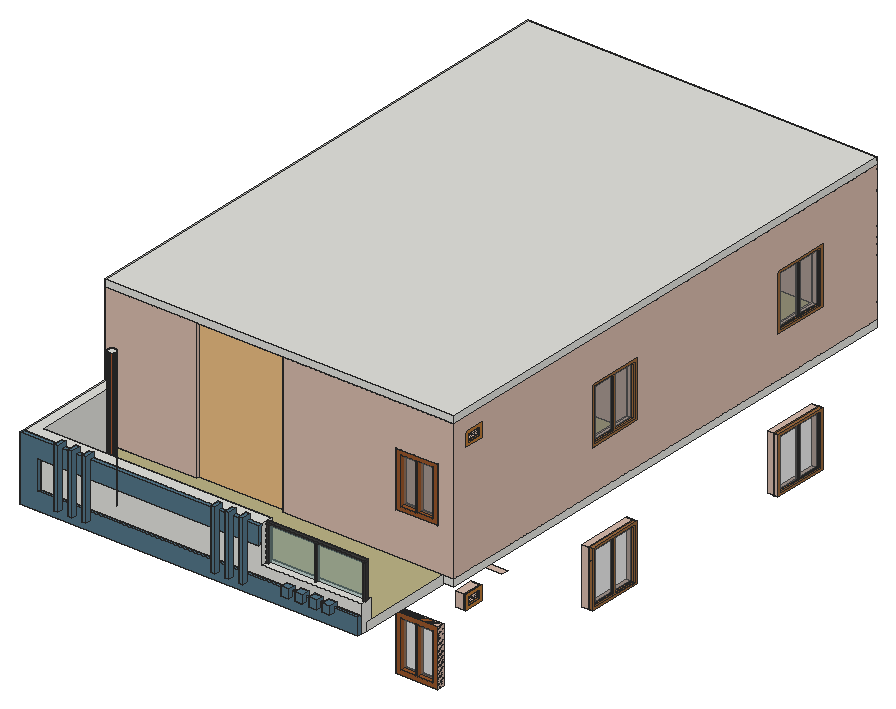
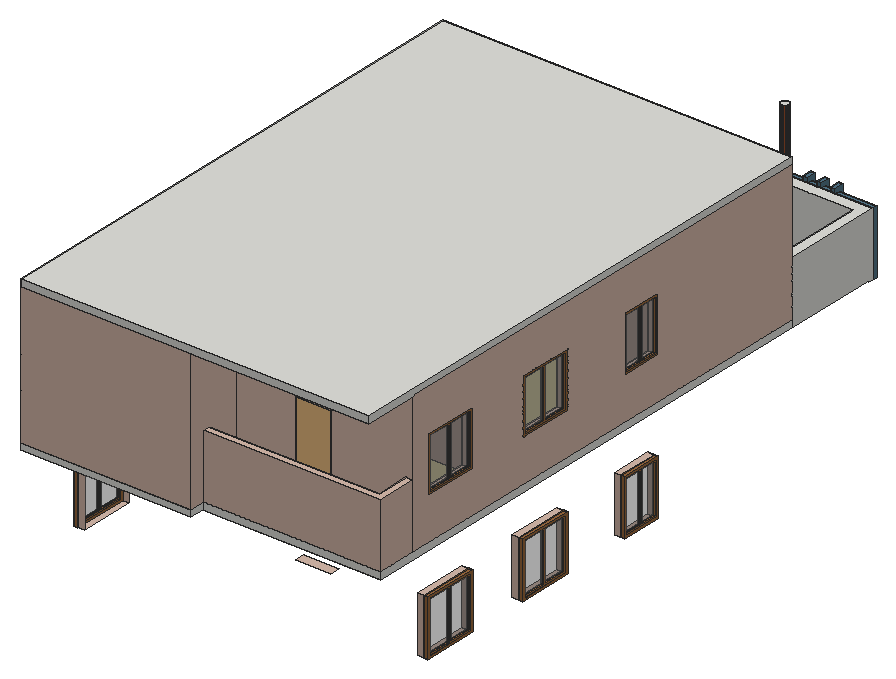
# SketchUp Ruby script. Lengths in inches.
U = 1.inch
M = Sketchup.active_model
def pt(a) = Geom::Point3d.new(a.map { |v| v * U })
def face(e, loops, mat)
  f = e.add_face(loops[0].map { |a| pt(a) })
  loops[1..].each { |l| e.add_face(l.map { |a| pt(a) }).erase! }
  f.material = f.back_material = mat if mat
  f
end
# faces: each face lists its corners as indices into pts; further lists are holes
def faces(e, pts, list, mat = nil) = list.each { |f| face(e, (f[0].is_a?(Array) ? f : [f]).map { |l| l.map { |i| pts[i] } }, mat) }
# xy, xz, yz: faces in a plane at the given z, y or x. An outline is a flat list of corners, or four numbers for a rectangle; further outlines are holes
def ring(l) = l.size == 4 ? [[l[0], l[1]], [l[2], l[1]], [l[2], l[3]], [l[0], l[3]]] : l.each_slice(2).to_a
def flat(e, list, mat, &to3) = list.each { |f| face(e, (f[0].is_a?(Array) ? f : [f]).map { |l| ring(l).map { |u, v| to3.(u, v) } }, mat) }
def xy(e, z, list, mat = nil) = flat(e, list, mat) { |x, y| [x, y, z] }
def xz(e, y, list, mat = nil) = flat(e, list, mat) { |x, z| [x, y, z] }
def yz(e, x, list, mat = nil) = flat(e, list, mat) { |y, z| [x, y, z] }
def lines(e, pts, list) = list.each { |a, b| e.add_line(pt(pts[a]), pt(pts[b])) }
# prism: a flat outline (further loops are holes) pulled along v
def prism(e, loops, v, mat = nil)
  f = face(e, loops, mat); d = Geom::Vector3d.new(v.map { |x| x * U })
  f.pushpull(f.normal.samedirection?(d) ? d.length : -d.length)
end
def box(e, o, s, mat = nil) = prism(e, [[o, [o[0] + s[0], o[1], o[2]], [o[0] + s[0], o[1] + s[1], o[2]], [o[0], o[1] + s[1], o[2]]]], [0, 0, s[2]], mat)
def at(x, y, z, deg = 0) = Geom::Transformation.translation(pt([x, y, z])) * Geom::Transformation.rotation(ORIGIN, Z_AXIS, deg.degrees)
def axes(o, x, y, z) = Geom::Transformation.new([*x, 0, *y, 0, *z, 0, *pt(o).to_a, 1])
def part(name) = M.definitions.add(name)
# library, detail: a bought-in or finely detailed component or shape, given as its bounding box
def library(name, o, s) = part(name).tap { |d| box(d.entities, o, s) }
def detail(e, o, s) = box(e.add_group.entities, o, s)
def put(e, d, t, mat = nil) = e.add_instance(d, t).tap { |i| i.material = mat if mat }
def group(e, t, mat = nil) = e.add_group.tap { |g| g.transformation = t; g.material = mat if mat }.entities
root = M.entities
M.materials.add("TEAKcrown-cut").color = [186, 122, 55]
M.materials.add("[0027_PeachPuff]").color = [83, 118, 137]
M.materials.add("[0042_Sienna]").color = [160, 82, 45]
M.materials.add("[Color B01]").color = [216, 187, 172]
M.materials.add("[Color E03]").color = [255, 255, 101]
M.materials.add("[Color E05]").color = [255, 255, 0]
M.materials.add("[Color M07]").color = [58, 58, 58]
M.materials.add("[Tile Ceramic Natural]").color = [189, 180, 134]
M.materials.add("[Translucent Glass Blue]").color = [141, 178, 174]
M.materials["[Translucent Glass Blue]"].alpha = 0.5
M.materials.add("[Translucent Glass Gray]").color = [128, 128, 128]
M.materials["[Translucent Glass Gray]"].alpha = 0.5
M.materials.add("[Translucent_Glass_Gray]3").color = [255, 255, 255]
M.materials["[Translucent_Glass_Gray]3"].alpha = 0.5
M.materials.add("[Wood Bamboo]").color = [122, 73, 29]
M.materials.add("[Wood Cherry Original]").color = [152, 86, 42]
M.materials.add("[Wood Floor]").color = [155, 105, 61]
c1 = part("window full")
xy(c1.entities,0,[[0,0,14.17,66.54]])
xy(c1.entities,2.26,[[12.2,2.26,14.17,64.28]],"[Wood Floor]")
xy(c1.entities,2.36,[[0,2.36,1.97,64.17]],"[Wood Floor]")
xy(c1.entities,3.74,[[11.42,3.74,12.2,32.875],[11.42,33.66,12.2,62.79]],"[Wood Floor]")
xy(c1.entities,3.9375,[[1.97,3.9375,2.76,32.77],[1.97,33.76,2.76,62.6]],"[Wood Floor]")
xy(c1.entities,4.18,[[2.76,4.18,11.42,32.09],[2.76,34.45,11.42,62.35]],"[Wood Floor]")
xy(c1.entities,69.83,[[2.76,4.18,11.42,32.09],[2.76,34.45,11.42,62.35]],"[Wood Floor]")
xy(c1.entities,70.08,[[1.97,3.9375,2.76,32.77],[1.97,33.76,2.76,62.6]])
xy(c1.entities,70.27,[[11.42,32.875,12.2,33.66]])
xy(c1.entities,70.27,[[11.42,3.74,12.2,32.875],[11.42,33.66,12.2,62.79]],"[Wood Floor]")
xy(c1.entities,71.65,[[0,2.36,1.97,64.17]])
xy(c1.entities,71.76,[[12.2,2.26,14.17,64.28]],"[Wood Floor]")
xy(c1.entities,74.02,[[0,0,14.17,66.54]],"[Wood Floor]")
xz(c1.entities,0,[[0,0,14.17,74.02]],"[Wood Floor]")
xz(c1.entities,2.26,[[12.2,2.26,14.17,71.76]],"[Wood Floor]")
xz(c1.entities,2.36,[[0,2.36,1.97,71.65]],"[Wood Floor]")
xz(c1.entities,3.74,[[11.42,3.74,12.2,70.27]],"[Wood Floor]")
xz(c1.entities,3.9375,[[1.97,3.9375,2.76,70.08]],"[Wood Floor]")
xz(c1.entities,4.18,[[2.76,4.18,11.42,69.83]],"[Wood Floor]")
xz(c1.entities,32.09,[[2.76,4.18,11.42,69.83]],"[Wood Floor]")
xz(c1.entities,32.77,[[1.97,3.9375,2.76,70.08]],"[Wood Floor]")
xz(c1.entities,32.875,[[11.42,3.74,12.2,70.27]],"[Wood Floor]")
xz(c1.entities,33.66,[[11.42,3.74,12.2,47.88],[11.42,47.88,12.2,70.27]],"[Wood Floor]")
xz(c1.entities,33.76,[[1.97,3.9375,2.76,70.08]],"[Wood Floor]")
xz(c1.entities,34.45,[[2.76,4.18,11.42,69.83]],"[Wood Floor]")
xz(c1.entities,62.35,[[2.76,4.18,11.42,69.83]],"[Wood Floor]")
xz(c1.entities,62.6,[[1.97,3.9375,2.76,70.08]],"[Wood Floor]")
xz(c1.entities,62.79,[[11.42,3.74,12.2,70.27]],"[Wood Floor]")
xz(c1.entities,64.17,[[0,2.36,1.97,71.65]],"[Wood Floor]")
xz(c1.entities,64.28,[[12.2,2.26,14.17,71.76]],"[Wood Floor]")
xz(c1.entities,66.54,[[0,0,14.17,74.02]],"[Wood Floor]")
yz(c1.entities,0,[[[0,0,66.54,74.02],[2.36,2.36,64.17,71.65]]],"[Wood Floor]")
yz(c1.entities,1.97,[[[2.36,2.36,64.17,71.65],[3.9375,3.9375,32.77,70.08],[33.76,3.9375,62.6,70.08]]],"[Wood Floor]")
yz(c1.entities,2.76,[[32.77,3.9375,33.76,4.18],[32.77,4.18,33.76,69.83],[32.77,69.83,33.76,70.08]])
yz(c1.entities,2.76,[[[3.9375,3.9375,32.77,70.08],[4.18,4.18,32.09,69.83]],[[33.76,3.9375,62.6,70.08],[34.45,4.18,62.35,69.83]]],"[Wood Floor]")
yz(c1.entities,11.42,[[32.875,69.83,33.66,70.27]])
yz(c1.entities,11.42,[[[3.74,3.74,32.875,70.27],[4.18,4.18,32.09,69.83]],[[33.66,3.74,62.79,70.27],[34.45,4.18,62.35,69.83]]],"[Wood Floor]")
yz(c1.entities,12.2,[[[2.26,2.26,64.28,71.76],[3.74,3.74,32.875,70.27],[33.66,3.74,62.79,70.27]]],"[Wood Floor]")
yz(c1.entities,14.17,[[[0,0,66.54,74.02],[2.26,2.26,64.28,71.76]]],"[Wood Floor]")
p = [[11.42,32.875,70.27],[11.42,32.875,70.28],[11.42,32.875,69.83],[11.42,32.09,69.83],[11.42,34.45,69.83],[11.42,33.66,69.83]]
lines(c1.entities,p,[[0,1],[2,3],[4,5]])
c2 = part("Group\#7")
g1 = group(c2.entities,at(1.67,3.02,2.71))
yz(g1,0,[[0,0,20.13,42.58]],"[Translucent Glass Gray]")
g2 = group(c2.entities,at(0,0,0))
put(g2,c1,axes([0,0,0],[0.2352,0,0],[0,0.72142,0],[0,0,0.64851]))
g3 = group(g2,at(1.67,24.85,2.71))
yz(g3,0,[[0,0,20.13,42.58]],"[Translucent Glass Gray]")
c3 = part("Group30\#1")
xy(c3.entities,0,[[-14.0625,-20.0625,-0.59,20.0625],[0.59,-20.0625,14.0625,20.0625]],"[Translucent Glass Gray]")
c4 = part("Group29\#1")
prism(c4.entities,[[[-18,24,0],[18,24,0],[18,-24,0],[-18,-24,0]],[[14.0625,20.0625,0],[0.59,20.0625,0],[0.59,-20.0625,0],[14.0625,-20.0625,0]],[[-0.59,20.0625,0],[-14.0625,20.0625,0],[-14.0625,-20.0625,0],[-0.59,-20.0625,0]]],[0,0,5.875],"[Wood Cherry Original]")
put(c4.entities,c3,at(0,0,2.9375))
c5 = part("Component\#10")
box(c5.entities,[0,0,0],[19,0.25,3.7],"[Translucent_Glass_Gray]3")
c6 = part("Ventilation_window")
g4 = group(c6.entities,at(-76.91,6.38,0),"TEAKcrown-cut")
xy(g4,-1.7,[[0,0,24,3]])
xy(g4,2.5,[[2.5,0,21.5,3]])
xy(g4,17.5,[[2.5,0,21.5,3]])
xy(g4,21.7,[[0,0,24,3]])
xz(g4,0,[[[0,-1.7,24,21.7],[2.5,2.5,21.5,17.5]]],"TEAKcrown-cut")
xz(g4,3,[[[0,-1.7,24,21.7],[2.5,2.5,21.5,17.5]]])
yz(g4,0,[[0,-1.7,3,21.7]])
yz(g4,2.5,[[0,2.5,3,2.5,3,4.31,0,6.48],[3,4.31,3,17.5,0,17.5,0,6.48]])
yz(g4,21.5,[[0,2.5,3,17.5]])
yz(g4,24,[[0,-1.7,3,21.7]])
put(g4,c5,axes([2.5,3.14,11.94],[1,0,0],[0,0.58779,0.80902],[0,-0.80902,0.58779]))
put(g4,c5,axes([2.5,3.16,14.6],[1,0,0],[0,0.58779,0.80902],[0,-0.80902,0.58779]))
put(g4,c5,axes([2.5,3,4.31],[1,0,0],[0,0.58779,0.80902],[0,-0.80902,0.58779]))
put(g4,c5,axes([2.5,3.14,9.46],[1,0,0],[0,0.58779,0.80902],[0,-0.80902,0.58779]))
put(g4,c5,axes([2.5,2.99,7.08],[1,0,0],[0,0.58779,0.80902],[0,-0.80902,0.58779]))
c7 = part("Group70\#1")
box(c7.entities,[313.8,73.72,268.25],[1.18,2.36,29.23])
c8 = part("Group69\#1")
box(c8.entities,[356.12,73.72,268.25],[2.36,2.36,29.23])
c9 = part("Group71\#1")
box(c9.entities,[270.3,73.52,297.48],[88.18,2.76,1.77])
c10 = part("Group68\#1")
box(c10.entities,[270.3,73.72,268.25],[2.37,2.36,29.23])
c11 = part("Group74\#1")
xz(c11.entities,74.9,[[271.49,268.25,357.3,297.48]],"[Translucent Glass Blue]")
c12 = part("Group\#12")
put(c12.entities,c7,at(-270.3,-73.52,-268.25),"[Color M07]")
put(c12.entities,c8,at(-270.3,-73.52,-268.25),"[Color M07]")
put(c12.entities,c9,at(-270.3,-73.52,-268.25),"[Color M07]")
put(c12.entities,c10,at(-270.3,-73.52,-268.25),"[Color M07]")
put(c12.entities,c11,at(-270.3,-73.52,-268.25))
c13 = part("Component\#9")
xy(c13.entities,0,[[[0,0,6.875,4],[0.7,0.7,6.17,3.3]]],"[Color E05]")
xy(c13.entities,0.625,[[0.7,0.7,6.17,3.3]],"[Color E05]")
xy(c13.entities,4.5625,[[0,4,6.875,6.6875]])
xy(c13.entities,7.25,[[0,0,6.875,6.6875]],"[0027_PeachPuff]")
xz(c13.entities,0,[[0,0,6.875,7.25]],"[0027_PeachPuff]")
xz(c13.entities,0.7,[[0.7,0,6.17,0.625]])
xz(c13.entities,3.3,[[0.7,0,6.17,0.625]],"[Color E05]")
xz(c13.entities,4,[[0,0,6.875,4.5625]])
xz(c13.entities,6.6875,[[0,4.5625,6.875,7.25]])
yz(c13.entities,0,[[0,0,0,7.25,6.6875,7.25,6.6875,4.5625,4,4.5625,4,0]],"[0027_PeachPuff]")
yz(c13.entities,0.7,[[0.7,0,3.3,0.625]],"[Color E05]")
yz(c13.entities,6.17,[[0.7,0,3.3,0.625]],"[Color E05]")
yz(c13.entities,6.875,[[0,0,4,0,4,4.5625,6.6875,4.5625,6.6875,7.25,0,7.25]],"[0027_PeachPuff]")
c14 = part("Vertical support post")
prism(c14.entities,[[[3.5625,0,-4],[3.5625,0,43.375],[3.5625,4,43.375],[3.5625,4,47.375],[3.5625,-4,47.375],[3.5625,-4,-4]]],[-3.5625,0,0],"[0027_PeachPuff]")
c15 = library("door by lz",[5.91,-4.92,0],[35.43,6.61,78.74])
c16 = part("Union")
xy(c16.entities,0,[[0,87.5,0,494.5,71.05,494.5,71.05,485.5,9,485.5,9,387.5,117,387.5,117,381.5,9,381.5,9,213.5,113.3,213.5,113.3,207.5,9,207.5,9,96.5,78.6875,96.5,78.6875,87.5],[[153,87.5,153,93.5,239,93.5,239,171.5,153,171.5,153,207.5,143.3,207.5,143.3,213.5,153,213.5,153,286.45,159,286.45,159,177.5,250.23,177.5,250.23,171.5,245,171.5,245,93.5,291,93.5,291,171.5,274.23,171.5,274.23,177.5,291,177.5,291,321.5,159,321.5,159,316.45,153,316.45,153,347.3125,159,347.3125,159,327.5,246,327.5,246,383.5,159,383.5,159,389.5,291,389.5,291,533.5,159,533.5,159,424.27,153,424.27,153,431.5,144.37,431.5,144.37,437.5,153,437.5,153,485.5,117,485.5,117,437.5,124.37,437.5,124.37,431.5,117,431.5,117,424.23,111,424.23,111,485.5,101.05,485.5,101.05,494.5,153,494.5,153,542.5,300,542.5,300,87.5],[252,327.5,291,383.5]],[153,377.3125,158.97,394.27],[111,387.5,117,394.27]])
xy(c16.entities,36,[[250.39,87.5,286.39,93.5],[0,230.6875,9,266.6875],[291,236.77,300,284.77],[0,328.61,9,376.61],[0,430.49,9,478.49],
  [291,436.51,300,484.51]])
xy(c16.entities,84,[[250.39,87.5,286.39,93.5],[250.23,171.5,274.23,177.5],[113.3,207.5,143.3,213.5],[0,230.6875,9,266.6875],[291,236.77,300,284.77],
  [153,286.45,159,316.45],[0,328.61,9,376.61],[153,347.3125,158.97,377.3125],[111,394.27,117,424.23],[153,394.27,159,424.27],
  [0,430.49,9,478.49],[124.37,431.5,144.37,437.5],[291,436.51,300,484.51],[71.05,485.5,101.05,494.5]])
xy(c16.entities,96,[[291,100.54,300,117.47]])
xy(c16.entities,108,[[291,100.54,300,117.47]])
xy(c16.entities,120,[[[0,87.5,78.6875,87.5,78.6875,96.5,9,96.5,9,207.5,153,207.5,153,171.5,239,171.5,239,93.5,153,93.5,153,87.5,300,87.5,300,542.5,153,542.5,153,494.5,0,494.5],[9,213.5,9,381.5,117,381.5,117,431.5,153,431.5,153,213.5],[159,327.5,159,347.3125,158.97,347.3125,158.97,394.27,159,394.27,159,533.5,291,533.5,291,389.5,159,389.5,159,383.5,246,383.5,246,327.5],[159,177.5,291,321.5],[9,387.5,111,485.5],[245,93.5,291,171.5],[252,327.5,291,383.5],[117,437.5,153,485.5]]])
xz(c16.entities,87.5,[[0,0,78.6875,120],[[153,0,300,120],[250.39,36,286.39,84]]],"[Color B01]")
xz(c16.entities,93.5,[[153,0,239,120],[[245,0,291,120],[250.39,36,286.39,84]]])
xz(c16.entities,96.5,[[9,0,78.6875,120]])
xz(c16.entities,100.54,[[291,96,300,108]])
xz(c16.entities,117.47,[[291,96,300,108]])
xz(c16.entities,171.5,[[153,0,239,120],[245,0,250.23,0,250.23,84,274.23,84,274.23,0,291,0,291,120,245,120]],"[Color B01]")
xz(c16.entities,177.5,[[159,0,159,120,291,120,291,0,274.23,0,274.23,84,250.23,84,250.23,0]])
xz(c16.entities,207.5,[[9,0,113.3,0,113.3,84,143.3,84,143.3,0,153,0,153,120,9,120]],"[Color B01]")
xz(c16.entities,213.5,[[9,0,113.3,120],[143.3,0,143.3,84,113.3,84,113.3,120,153,120,153,0]])
xz(c16.entities,230.6875,[[0,36,9,84]])
xz(c16.entities,236.77,[[291,36,300,84]])
xz(c16.entities,266.6875,[[0,36,9,84]])
xz(c16.entities,284.77,[[291,36,300,84]])
xz(c16.entities,286.45,[[153,0,159,84]])
xz(c16.entities,316.45,[[153,0,159,84]])
xz(c16.entities,321.5,[[159,0,291,120]],"[Color B01]")
xz(c16.entities,327.5,[[159,0,246,120],[252,0,291,120]])
xz(c16.entities,328.61,[[0,36,9,84]])
xz(c16.entities,347.3125,[[153,0,153,84,158.97,84,158.97,120,159,120,159,0]])
xz(c16.entities,376.61,[[0,36,9,84]])
xz(c16.entities,377.3125,[[153,0,158.97,84]])
xz(c16.entities,381.5,[[9,0,117,120]],"[Color B01]")
xz(c16.entities,383.5,[[252,0,291,120]])
xz(c16.entities,383.5,[[159,0,246,120]],"[Color B01]")
xz(c16.entities,387.5,[[9,0,111,120]])
xz(c16.entities,389.5,[[159,0,291,120]])
xz(c16.entities,394.27,[[111,0,117,84],[153,0,158.97,84],[158.97,84,159,120]])
xz(c16.entities,424.23,[[111,0,117,84]])
xz(c16.entities,424.27,[[153,0,159,84]])
xz(c16.entities,430.49,[[0,36,9,84]])
xz(c16.entities,431.5,[[117,0,124.37,0,124.37,84,144.37,84,144.37,0,153,0,153,120,117,120]],"[Color B01]")
xz(c16.entities,436.51,[[291,36,300,84]])
xz(c16.entities,437.5,[[117,0,117,120,153,120,153,0,144.37,0,144.37,84,124.37,84,124.37,0]])
xz(c16.entities,478.49,[[0,36,9,84]])
xz(c16.entities,484.51,[[291,36,300,84]])
xz(c16.entities,485.5,[[117,0,153,120]])
xz(c16.entities,485.5,[[9,0,71.05,0,71.05,84,101.05,84,101.05,0,111,0,111,120,9,120]],"[Color B01]")
xz(c16.entities,494.5,[[0,0,0,120,153,120,153,0,101.05,0,101.05,84,71.05,84,71.05,0]])
xz(c16.entities,533.5,[[159,0,291,120]],"[Color B01]")
xz(c16.entities,542.5,[[153,0,300,120]])
yz(c16.entities,0,[[[87.5,0,494.5,120],[430.49,36,478.49,84],[328.61,36,376.61,84],[230.6875,36,266.6875,84]]],"[Color B01]")
yz(c16.entities,9,[[96.5,0,207.5,120],[[213.5,0,381.5,120],[328.61,36,376.61,84],[230.6875,36,266.6875,84]],[[387.5,0,485.5,120],[430.49,36,478.49,84]]])
yz(c16.entities,71.05,[[485.5,0,494.5,84]])
yz(c16.entities,78.6875,[[87.5,0,96.5,120]])
yz(c16.entities,101.05,[[485.5,0,494.5,84]])
yz(c16.entities,111,[[387.5,0,387.5,120,485.5,120,485.5,0,424.23,0,424.23,84,394.27,84,394.27,0]])
yz(c16.entities,113.3,[[207.5,0,213.5,84]])
yz(c16.entities,117,[[381.5,0,394.27,0,394.27,84,424.23,84,424.23,0,431.5,0,431.5,120,381.5,120],[437.5,0,485.5,120]])
yz(c16.entities,124.37,[[431.5,0,437.5,84]])
yz(c16.entities,143.3,[[207.5,0,213.5,84]])
yz(c16.entities,144.37,[[431.5,0,437.5,84]])
yz(c16.entities,153,[[87.5,0,93.5,120],[437.5,0,485.5,120],[494.5,0,542.5,120]])
yz(c16.entities,153,[[171.5,0,207.5,120],[213.5,0,213.5,120,431.5,120,431.5,0,424.27,0,424.27,84,394.27,84,394.27,0,377.3125,0,377.3125,84,347.3125,84,347.3125,0,316.45,0,316.45,84,286.45,84,286.45,0]],"[Color B01]")
yz(c16.entities,158.97,[[377.3125,0,394.27,0,394.27,120,347.3125,120,347.3125,84,377.3125,84]])
yz(c16.entities,159,[[327.5,0,347.3125,120],[383.5,0,389.5,120],[424.27,0,533.5,0,533.5,120,394.27,120,394.27,84,424.27,84]])
yz(c16.entities,159,[[177.5,0,286.45,0,286.45,84,316.45,84,316.45,0,321.5,0,321.5,120,177.5,120]],"[Color B01]")
yz(c16.entities,239,[[93.5,0,171.5,120]])
yz(c16.entities,245,[[93.5,0,171.5,120]])
yz(c16.entities,246,[[327.5,0,383.5,120]])
yz(c16.entities,250.23,[[171.5,0,177.5,84]])
yz(c16.entities,250.39,[[87.5,36,93.5,84]])
yz(c16.entities,252,[[327.5,0,383.5,120]])
yz(c16.entities,274.23,[[171.5,0,177.5,84]])
yz(c16.entities,286.39,[[87.5,36,93.5,84]])
yz(c16.entities,291,[[[93.5,0,171.5,120],[100.54,96,117.47,108]],[[177.5,0,321.5,120],[236.77,36,284.77,84]],[327.5,0,383.5,120],[[389.5,0,533.5,120],[436.51,36,484.51,84]]])
yz(c16.entities,300,[[[87.5,0,542.5,120],[436.51,36,484.51,84],[236.77,36,284.77,84],[100.54,96,117.47,108]]],"[Color B01]")
put(c16.entities,c15,axes([153.59,321.46,0],[0,-0.84667,0],[0.14881,0,0],[0,0,1.0668]))
put(c16.entities,c15,axes([153.59,382.32,0],[0,-0.84667,0],[0.14881,0,0],[0,0,1.0668]))
put(c16.entities,c15,axes([153.59,429.27,0],[0,-0.84667,0],[0.14881,0,0],[0,0,1.0668]))
put(c16.entities,c15,axes([116.41,429.27,0],[0,-0.84667,0],[-0.14881,0,0],[0,0,1.0668]))
put(c16.entities,c15,axes([108.3,208.09,0],[0.84667,0,0],[0,0.14881,0],[0,0,1.0668]))
put(c16.entities,c15,axes([246.23,177.5,0],[0.67733,0,0],[0,0.14881,0],[0,0,1.0668]))
put(c16.entities,c15,axes([66.05,494.59,0],[0.84667,0,0],[0,0.14881,0],[0,0,1.0668]))
put(c16.entities,c6,axes([303.45,154.81,96.87],[0,0.70573,0],[-0.54,0,0],[0,0,0.51282]))
put(c16.entities,c2,at(0,328.61,36))
put(c16.entities,c2,at(0,430.49,36))
put(c16.entities,c2,at(296.67,436.51,36))
put(c16.entities,c2,at(296.67,236.77,36))
put(c16.entities,c2,axes([0,230.6875,36],[1,0,0],[0,0.75,0],[0,0,1]))
put(c16.entities,c4,axes([268.39,93.375,60],[1,0,0],[0,0,1],[0,-1,0]))
c17 = part("Union\#1")
prism(c17.entities,[[[153,29,0],[6,29,0],[6,0,0],[0,0,0],[0,35,0],[153,35,0]]],[0,0,55.4375])
c18 = library("Sliding Door (1.93 x 2.21)",[0,-1.25,-0.01],[76.06,6.25,87.01])
xy(root,191.75,[[250.39,134.5,286.39,140.5],[0,277.6875,9,313.6875],[291,283.77,300,331.77],[0,375.61,9,423.61],[0,477.49,9,525.49],
  [291,483.51,300,531.51]],"[Color B01]")
xy(root,239.75,[[250.39,134.5,286.39,140.5],[250.23,218.5,274.23,224.5],[113.3,254.5,143.3,260.5],[0,277.6875,9,313.6875],[291,283.77,300,331.77],
  [153,333.45,159,363.45],[0,375.61,9,423.61],[153,394.3125,158.97,424.3125],[111,441.27,117,471.23],[153,441.27,159,471.27],
  [0,477.49,9,525.49],[124.37,478.5,144.37,484.5],[291,483.51,300,531.51],[71.05,532.5,101.05,541.5]],"[Color B01]")
xy(root,251.75,[[291,147.54,300,164.47]],"[Color B01]")
xy(root,263.75,[[291,147.54,300,164.47]],"[Color B01]")
xy(root,275.75,[[[0,134.5,78.6875,134.5,78.6875,140.5,9,140.5,9,254.5,153,254.5,153,218.5,239,218.5,239,140.5,153,140.5,153,134.5,300,134.5,300,589.5,153,589.5,153,541.5,0,541.5],[9,260.5,9,428.5,117,428.5,117,478.5,153,478.5,153,260.5],[159,374.5,159,394.3125,158.97,394.3125,158.97,441.27,159,441.27,159,580.5,291,580.5,291,436.5,159,436.5,159,430.5,246,430.5,246,374.5],[159,224.5,291,368.5],[9,434.5,111,532.5],[245,140.5,291,218.5],[252,374.5,291,430.5],[117,484.5,153,532.5]]],"[Color B01]")
xy(root,281.75,[[57.2,66.45,56.26,66.57,55.38,66.93,54.63,67.51,54.06,68.26,53.69,69.14,53.57,70.07,53.69,71.01,54.06,71.89,54.63,72.64,55.38,73.21,56.26,73.58,57.2,73.7,58.13,73.58,59.01,73.21,59.76,72.64,60.34,71.89,60.7,71.01,60.82,70.07,60.7,69.14,60.34,68.26,59.76,67.51,59.01,66.93,58.13,66.57]])
xy(root,400.875,[[57.2,66.45,58.13,66.57,59.01,66.93,59.76,67.51,60.34,68.26,60.7,69.14,60.82,70.07,60.7,71.01,60.34,71.89,59.76,72.64,59.01,73.21,58.13,73.58,57.2,73.7,56.26,73.58,55.38,73.21,54.63,72.64,54.06,71.89,53.69,71.01,53.57,70.07,53.69,69.14,54.06,68.26,54.63,67.51,55.38,66.93,56.26,66.57]])
xz(root,147.54,[[291,251.75,300,263.75]],"[Color B01]")
xz(root,164.47,[[291,251.75,300,263.75]],"[Color B01]")
xz(root,277.6875,[[0,191.75,9,239.75]],"[Color B01]")
xz(root,283.77,[[291,191.75,300,239.75]],"[Color B01]")
xz(root,313.6875,[[0,191.75,9,239.75]],"[Color B01]")
xz(root,331.77,[[291,191.75,300,239.75]],"[Color B01]")
xz(root,375.61,[[0,191.75,9,239.75]],"[Color B01]")
xz(root,423.61,[[0,191.75,9,239.75]],"[Color B01]")
xz(root,441.27,[[158.97,239.75,159,275.75]],"[Color B01]")
xz(root,477.49,[[0,191.75,9,239.75]],"[Color B01]")
xz(root,483.51,[[291,191.75,300,239.75]],"[Color B01]")
xz(root,525.49,[[0,191.75,9,239.75]],"[Color B01]")
xz(root,531.51,[[291,191.75,300,239.75]],"[Color B01]")
yz(root,250.39,[[134.5,191.75,140.5,239.75]],"[Color B01]")
yz(root,286.39,[[134.5,191.75,140.5,239.75]],"[Color B01]")
p = [[56.26,66.57,281.75],[57.2,66.45,281.75],[57.2,66.45,400.875],[56.26,66.57,400.875],[58.13,66.57,281.75],[58.13,66.57,400.875],
  [55.38,66.93,281.75],[55.38,66.93,400.875],[59.01,66.93,281.75],[59.01,66.93,400.875],[54.63,67.51,281.75],[54.63,67.51,400.875],
  [59.76,67.51,281.75],[59.76,67.51,400.875],[54.06,68.26,281.75],[54.06,68.26,400.875],[60.34,68.26,281.75],[60.34,68.26,400.875],
  [53.69,69.14,281.75],[53.69,69.14,400.875],[60.7,69.14,281.75],[60.7,69.14,400.875],[53.57,70.07,281.75],[53.57,70.07,400.875],
  [60.82,70.07,281.75],[60.82,70.07,400.875],[53.69,71.01,281.75],[53.69,71.01,400.875],[60.7,71.01,281.75],[60.7,71.01,400.875],
  [54.06,71.89,281.75],[54.06,71.89,400.875],[60.34,71.89,281.75],[60.34,71.89,400.875],[54.63,72.64,281.75],[54.63,72.64,400.875],
  [59.76,72.64,281.75],[59.76,72.64,400.875],[55.38,73.21,281.75],[55.38,73.21,400.875],[59.01,73.21,281.75],[59.01,73.21,400.875],
  [56.26,73.58,281.75],[56.26,73.58,400.875],[58.13,73.58,281.75],[58.13,73.58,400.875],[57.2,73.7,281.75],[57.2,73.7,400.875]]
faces(root,p,[[0,1,2,3],[1,4,5,2],[6,0,3,7],[4,8,9,5],[10,6,7,11],[8,12,13,9],[14,10,11,15],[12,16,17,13],
  [18,14,15,19],[16,20,21,17],[22,18,19,23],[20,24,25,21],[26,22,23,27],[24,28,29,25],[30,26,27,31],[28,32,33,29],
  [34,30,31,35],[32,36,37,33],[38,34,35,39],[36,40,41,37],[42,38,39,43],[40,44,45,41],[46,42,43,47],[44,46,47,45]],"[0042_Sienna]")
put(root,c2,axes([0,277.6875,191.75],[1,0,0],[0,0.75,0],[0,0,1]),"[Color B01]")
put(root,c2,at(296.67,483.51,191.75),"[Color B01]")
put(root,c2,at(296.67,283.77,191.75),"[Color B01]")
put(root,c2,at(0,477.49,191.75),"[Color B01]")
put(root,c2,at(0,375.61,191.75),"[Color B01]")
put(root,c4,axes([268.39,140.375,215.75],[1,0,0],[0,0,1],[0,-1,0]),"[Color B01]")
put(root,c6,axes([303.45,201.81,252.62],[0,0.70573,0],[-0.54,0,0],[0,0,0.51282]),"[Color B01]")
g5 = group(root,at(0,47,275.75))
xy(g5,-1.5625,[[[4,4,291,87.5],[6,6,289,85.5]]],"[Wood Cherry Original]")
xy(g5,0,[[0,87.5,0,529.5,153,529.5,153,542.5,300,542.5,300,87.5]])
xy(g5,0,[[6,6,289,85.5]],"[Wood Bamboo]")
xy(g5,6,[[4,4,291,4,291,87.5,300,87.5,300,542.5,153,542.5,153,529.5,0,529.5,0,87.5,4,87.5]],"[Tile Ceramic Natural]")
xz(g5,4,[[4,-1.5625,291,6]],"[Wood Cherry Original]")
xz(g5,6,[[6,-1.5625,289,0]])
xz(g5,85.5,[[6,-1.5625,289,0]],"[Wood Cherry Original]")
xz(g5,87.5,[[4,-1.5625,291,0],[0,0,4,6],[291,0,300,6]])
xz(g5,529.5,[[0,0,153,6]])
xz(g5,542.5,[[153,0,300,6]])
yz(g5,0,[[87.5,0,529.5,6]])
yz(g5,4,[[4,-1.5625,87.5,6]],"[Wood Cherry Original]")
yz(g5,6,[[6,-1.5625,85.5,0]],"[Wood Cherry Original]")
yz(g5,153,[[529.5,0,542.5,6]])
yz(g5,289,[[6,-1.5625,85.5,0]],"[Wood Cherry Original]")
yz(g5,291,[[4,-1.5625,87.5,6]])
yz(g5,300,[[87.5,0,542.5,6]])
g6 = group(root,at(0,39,274.5625))
put(g6,c12,axes([205.1875,11.62,23.4375],[0.97321,0,0],[0,1,0],[0,0,1.02]))
g7 = group(g6,at(0,0,0))
put(g7,c13,at(251.27,0,10.78))
put(g7,c13,at(239.27,0,10.78))
put(g7,c13,at(263.27,0,10.78))
put(g7,c13,at(227.27,0,10.78))
g8 = group(g7,at(0,0,0))
put(g8,c14,at(179.125,4,11.8125))
put(g8,c14,at(167.125,4,11.8125))
put(g8,c14,at(191.125,4,11.8125))
put(g8,c14,at(56.1875,4,11.8125))
put(g8,c14,at(32.1875,4,11.8125))
put(g8,c14,at(44.1875,4,11.8125))
g9 = group(g8,at(0,12,7.1875))
xy(g9,-7.1875,[[0,-4,291,0]])
xy(g9,-7.1875,[[0,-8,291,-4]],"[0027_PeachPuff]")
xy(g9,-6,[[0,0,4,83.5]])
xy(g9,0,[[4,0,4,83.5,9,83.5,9,6,291,6,291,0]])
xy(g9,7.1,[[14.78,-6.5,291,-4]],"[Color E03]")
xy(g9,8.16,[[15.35,-8,291,-6.5]],"[0027_PeachPuff]")
xy(g9,16.25,[[205.1875,-4,291,6]])
xy(g9,32.65,[[15.35,-8,205.1875,-6.5]],"[0027_PeachPuff]")
xy(g9,33.97,[[14.78,-6.5,205.1875,-4]],"[Color E03]")
xy(g9,48,[[0,-4,205.1875,-4,205.1875,6,9,6,9,83.5,0,83.5]])
xy(g9,48,[[0,-8,205.1875,-4]],"[0027_PeachPuff]")
xz(g9,-8,[[0,-7.1875,291,-7.1875,291,8.16,15.35,8.16,15.35,32.65,205.1875,32.65,205.1875,48,0,48]],"[0027_PeachPuff]")
xz(g9,-6.5,[[14.78,7.1,291,8.16],[14.78,8.16,15.35,33.97],[15.35,32.65,205.1875,33.97]])
xz(g9,-4,[[0,-7.1875,0,48,205.1875,48,205.1875,33.97,14.78,33.97,14.78,7.1,291,7.1,291,-7.1875],[14.78,7.1,291,7.1,291,16.25,205.1875,16.25,205.1875,33.97,14.78,33.97]])
xz(g9,0,[[0,-7.1875,4,-6],[4,-7.1875,291,0]])
xz(g9,6,[[9,0,9,48,205.1875,48,205.1875,16.25,291,16.25,291,0]])
xz(g9,83.5,[[0,-6,0,48,9,48,9,0,4,0,4,-6]])
yz(g9,0,[[-4,-7.1875,-4,48,83.5,48,83.5,-6,0,-6,0,-7.1875]])
yz(g9,0,[[-8,-7.1875,-4,48]],"[0027_PeachPuff]")
yz(g9,4,[[0,-6,83.5,0]])
yz(g9,9,[[6,0,83.5,48]])
yz(g9,14.78,[[-6.5,7.1,-4,33.97]],"[Color E03]")
yz(g9,15.35,[[-8,8.16,-6.5,32.65]],"[0027_PeachPuff]")
yz(g9,205.1875,[[-4,16.25,6,48]])
yz(g9,205.1875,[[-8,32.65,-6.5,32.65,-6.5,33.97,-4,33.97,-4,48,-8,48]],"[0027_PeachPuff]")
yz(g9,291,[[-4,-7.1875,0,-7.1875,0,0,6,0,6,16.25,-4,16.25]])
yz(g9,291,[[-8,-7.1875,-4,-7.1875,-4,7.1,-6.5,7.1,-6.5,8.16,-8,8.16]],"[0027_PeachPuff]")
put(root,c16,at(0,47,281.75),"[Color B01]")
put(root,c17,at(0,541.5,281.75),"[Color B01]")
put(root,c18,axes([78.6875,137.2,282.38],[1,0,0],[0,0.71,0],[0,0,1.37927]),"[Wood Cherry Original]")
g10 = group(root,at(0,47,401.75))
box(g10,[0,87.5,0],[300,455,6])
